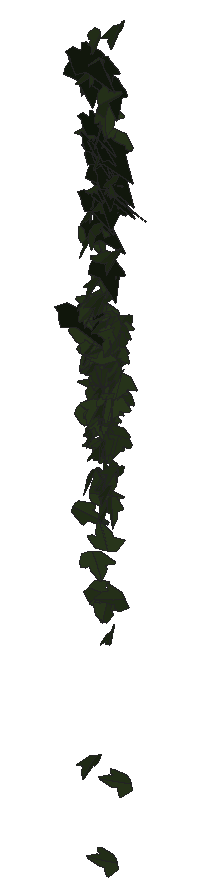
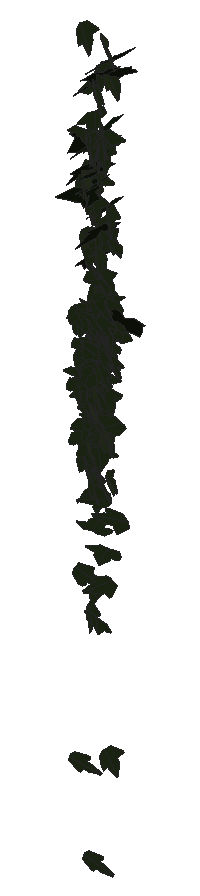
# SketchUp Ruby script. Lengths in inches.
U = 1.inch
M = Sketchup.active_model
def pt(a) = Geom::Point3d.new(a.map { |v| v * U })
def face(e, loops, mat)
  f = e.add_face(loops[0].map { |a| pt(a) })
  loops[1..].each { |l| e.add_face(l.map { |a| pt(a) }).erase! }
  f.material = f.back_material = mat if mat
  f
end
# faces: each face lists its corners as indices into pts; further lists are holes
def faces(e, pts, list, mat = nil) = list.each { |f| face(e, (f[0].is_a?(Array) ? f : [f]).map { |l| l.map { |i| pts[i] } }, mat) }
# xy, xz, yz: faces in a plane at the given z, y or x. An outline is a flat list of corners, or four numbers for a rectangle; further outlines are holes
def ring(l) = l.size == 4 ? [[l[0], l[1]], [l[2], l[1]], [l[2], l[3]], [l[0], l[3]]] : l.each_slice(2).to_a
def flat(e, list, mat, &to3) = list.each { |f| face(e, (f[0].is_a?(Array) ? f : [f]).map { |l| ring(l).map { |u, v| to3.(u, v) } }, mat) }
def xy(e, z, list, mat = nil) = flat(e, list, mat) { |x, y| [x, y, z] }
def xz(e, y, list, mat = nil) = flat(e, list, mat) { |x, z| [x, y, z] }
def yz(e, x, list, mat = nil) = flat(e, list, mat) { |y, z| [x, y, z] }
def lines(e, pts, list) = list.each { |a, b| e.add_line(pt(pts[a]), pt(pts[b])) }
# prism: a flat outline (further loops are holes) pulled along v
def prism(e, loops, v, mat = nil)
  f = face(e, loops, mat); d = Geom::Vector3d.new(v.map { |x| x * U })
  f.pushpull(f.normal.samedirection?(d) ? d.length : -d.length)
end
def box(e, o, s, mat = nil) = prism(e, [[o, [o[0] + s[0], o[1], o[2]], [o[0] + s[0], o[1] + s[1], o[2]], [o[0], o[1] + s[1], o[2]]]], [0, 0, s[2]], mat)
def at(x, y, z, deg = 0) = Geom::Transformation.translation(pt([x, y, z])) * Geom::Transformation.rotation(ORIGIN, Z_AXIS, deg.degrees)
def axes(o, x, y, z) = Geom::Transformation.new([*x, 0, *y, 0, *z, 0, *pt(o).to_a, 1])
def part(name) = M.definitions.add(name)
# library, detail: a bought-in or finely detailed component or shape, given as its bounding box
def library(name, o, s) = part(name).tap { |d| box(d.entities, o, s) }
def detail(e, o, s) = box(e.add_group.entities, o, s)
def put(e, d, t, mat = nil) = e.add_instance(d, t).tap { |i| i.material = mat if mat }
def group(e, t, mat = nil) = e.add_group.tap { |g| g.transformation = t; g.material = mat if mat }.entities
root = M.entities
M.materials.add("1026 AP 7946 SUNNY SIDE UP").color = [254, 231, 186]
M.materials.add("efeu1").color = [18, 25, 13]
M.materials.add("efeu2").color = [43, 57, 29]
c1 = part("ivyleaf_9")
p = [[1.54,2.16,1.25],[1.36,2.04,1.19],[-0.21,0.99,0.68],[-0.71,1.11,0.82],[-0.85,0.86,0.67],[-0.8,0.17,0.21],
  [-0.9,-0.01,0.1],[-0.67,-0.16,-0.02],[-0.08,-0.08,-0.05],[-0.03,-0.6,-0.4],[0.65,-0.88,-0.66],[0.83,-0.6,-0.49],
  [1.29,-0.42,-0.43],[1.8125,-0.07,-0.26],[1.21,0.44,0.15]]
faces(c1.entities,p,[[0,1,2,3,4,5,6,7,8,9,10,11,12,13,14]],"efeu1")
c2 = part("ivyleaf_10")
p = [[0,0.5,-0.03],[-0.0625,2.02,-0.43],[-0.19,2.01,-0.46],[-0.54,1.05,-0.29],[-0.52,0.625,-0.18],[-0.83,0.76,-0.28],
  [-1.16,0.64,-0.33],[-1.15,0.33,-0.24],[-0.77,-0.39,0.02],[-0.3,-0.51,0.16],[0.04,-0.48,0.23],[-0.02,2.01,-0.4375],
  [-0.06,2.01,-0.43],[0.04,-0.49,0.23],[0.67,-0.49,0.14],[1.38,0.36,-0.2],[1.375,0.51,-0.24],[0.81,0.65,-0.19],
  [0.62,0.59,-0.15],[0.6,1.09,-0.28],[0.5,1.23,-0.31]]
faces(c2.entities,p,[[0,1,2,3,4,5,6,7,8,9,10],[11,12,0,13,14,15,16,17,18,19,20]],"efeu2")
put(root,c1,axes([104.51,212.62,261.08],[-0.10189,-0.126,-0.22492],[0.26137,0.14715,-0.1379],[0.29668,-0.17291,0.04425]),"1026 AP 7946 SUNNY SIDE UP")
put(root,c2,axes([104.8,212.79,260.43],[0.14788,-0.18919,-0.06949],[-0.05325,0.05728,-0.21727],[0.31074,0.09986,-0.00416]),"1026 AP 7946 SUNNY SIDE UP")
put(root,c2,axes([104.78,212.86,258.33],[0.02808,-0.20182,0.05139],[-0.00344,-0.0514,-0.20892],[0.32731,0.01677,-0.00661]),"1026 AP 7946 SUNNY SIDE UP")
put(root,c2,axes([104.79,212.68,263.45],[0.03722,-0.22123,-0.10419],[-0.00875,0.09983,-0.22858],[0.38157,0.02387,0.00492]),"1026 AP 7946 SUNNY SIDE UP")
put(root,c2,axes([104.56,212.83,258.71],[0.15363,0.1008,0.18602],[0.18817,0.13453,-0.14375],[-0.26422,0.15442,0.00578]),"1026 AP 7946 SUNNY SIDE UP")
put(root,c2,axes([104.85,212.91,259.35],[-0.24055,-0.1247,0.08015],[-0.06584,-0.07172,-0.20183],[0.22216,-0.15628,0.02697]),"1026 AP 7946 SUNNY SIDE UP")
put(root,c2,axes([104.52,212.71,256.46],[-0.07971,-0.01702,-0.21016],[0.31895,-0.03174,-0.04941],[-0.04221,-0.2077,0.02353]),"1026 AP 7946 SUNNY SIDE UP")
put(root,c2,axes([104.81,212.76,260.13],[0.30669,-0.08194,-0.05742],[-0.09193,0.00295,-0.21702],[0.12532,0.2027,-0.01868]),"1026 AP 7946 SUNNY SIDE UP")
put(root,c2,axes([104.8125,212.65,266.57],[0.01044,-0.25506,0.02697],[-0.0004,-0.02764,-0.26301],[0.4034,0.00657,-0.00096]),"1026 AP 7946 SUNNY SIDE UP")
put(root,c2,axes([104.74,212.76,257.33],[0.11427,-0.15771,0.10792],[0.06501,-0.09726,-0.17944],[0.29132,0.08357,-0.00229]),"1026 AP 7946 SUNNY SIDE UP")
put(root,c2,axes([104.8,212.85,264.95],[0.0122,-0.23605,-0.05486],[0.0232,0.0523,-0.24244],[0.37933,0.00439,0.01659]),"1026 AP 7946 SUNNY SIDE UP")
put(root,c2,axes([104.79,212.67,262.84],[0.1113,-0.21199,0.07766],[0.02038,-0.07632,-0.2304],[0.35384,0.07108,-0.01116]),"1026 AP 7946 SUNNY SIDE UP")
put(root,c2,axes([104.83,212.74,258.55],[0.0412,-0.21263,-0.05682],[-0.02422,0.05241,-0.22022],[0.34408,0.02915,-0.0087]),"1026 AP 7946 SUNNY SIDE UP")
put(root,c2,axes([104.84,212.78,260.92],[0.22749,-0.13987,-0.09949],[-0.06758,0.09154,-0.20406],[0.25784,0.14739,0.03429]),"1026 AP 7946 SUNNY SIDE UP")
put(root,c2,axes([104.83,212.9,259.9],[-0.01707,-0.21632,0.02637],[0.00079,-0.02688,-0.22328],[0.34275,-0.01071,0.00183]),"1026 AP 7946 SUNNY SIDE UP")
put(root,c2,axes([104.91,212.97,259.98],[-0.30974,0.06925,0.05127],[-0.11245,-0.06746,-0.19686],[-0.07238,-0.19154,0.08646]),"1026 AP 7946 SUNNY SIDE UP")
put(root,c2,axes([104.82,212.81,267.33],[0.21445,-0.21888,-0.00563],[-0.01642,-0.00153,-0.2655],[0.34384,0.13644,-0.00916]),"1026 AP 7946 SUNNY SIDE UP")
put(root,c2,axes([104.89,212.73,261.34],[-0.14405,-0.16021,0.15164],[-0.034,-0.15318,-0.18537],[0.34138,-0.08286,0.04552]),"1026 AP 7946 SUNNY SIDE UP")
put(root,c2,axes([104.87,212.85,265.2],[-0.23667,-0.19164,0.0436],[0.00181,-0.05555,-0.24881],[0.30897,-0.14647,0.03486]),"1026 AP 7946 SUNNY SIDE UP")
put(root,c1,axes([104.72,212.6875,266.68],[-0.10214,-0.24221,-0.0535],[0.03916,0.04561,-0.25778],[0.38709,-0.06853,0.01196]),"1026 AP 7946 SUNNY SIDE UP")
put(root,c2,axes([104.875,212.9,259.69],[-0.22992,-0.14841,0.05033],[-0.00212,-0.06681,-0.21002],[0.24608,-0.13923,0.04521]),"1026 AP 7946 SUNNY SIDE UP")
put(root,c2,axes([104.85,212.67,260.38],[0.09904,-0.21439,0.04253],[0.00216,-0.04384,-0.23018],[0.34366,0.06206,-0.01081]),"1026 AP 7946 SUNNY SIDE UP")
put(root,c2,axes([104.74,213.15,254.29],[0.30393,-0.05318,0.06214],[0.08204,-0.03757,-0.20556],[0.09669,0.19906,-0.02091]),"1026 AP 7946 SUNNY SIDE UP")
put(root,c2,axes([104.88,212.64,250.91],[-0.04262,-0.21887,0.0626],[-0.01019,-0.06167,-0.22756],[0.35755,-0.02785,0.00097]),"1026 AP 7946 SUNNY SIDE UP")
put(root,c2,axes([104.83,212.73,261.375],[-0.13025,-0.20028,-0.08539],[0.0714,0.06949,-0.22238],[0.33256,-0.09336,0.0143]),"1026 AP 7946 SUNNY SIDE UP")
put(root,c2,axes([104.875,212.86,257.29],[0.18386,-0.17254,-0.02444],[-0.03716,0.0114,-0.21423],[0.27111,0.11857,-0.0128]),"1026 AP 7946 SUNNY SIDE UP")
put(root,c2,axes([104.875,212.62,261.21],[0.13267,-0.21299,-0.00805],[-0.01159,0.00418,-0.23592],[0.33486,0.08453,-0.00498]),"1026 AP 7946 SUNNY SIDE UP")
put(root,c2,axes([104.65,212.83,260.875],[0.2714,0.02668,0.13493],[0.20861,-0.01031,-0.17823],[-0.02353,0.21633,-0.02385]),"1026 AP 7946 SUNNY SIDE UP")
put(root,c2,axes([104.86,212.95,258.01],[-0.20099,-0.15647,0.02288],[0.04302,-0.05113,-0.2011],[0.24495,-0.11941,0.0541]),"1026 AP 7946 SUNNY SIDE UP")
put(root,c2,axes([104.8,212.77,258.53],[-0.05877,-0.11426,-0.19811],[0.11385,0.1776,-0.12259],[0.33187,-0.08116,0.00697]),"1026 AP 7946 SUNNY SIDE UP")
put(root,c2,axes([104.59,212.58,260.71],[0.13878,0.03307,0.21578],[0.32198,0.04486,-0.09601],[-0.08549,0.22264,-0.01132]),"1026 AP 7946 SUNNY SIDE UP")
put(root,c2,axes([104.89,212.91,260.31],[0.24752,-0.13403,-0.06789],[-0.05479,0.05902,-0.21151],[0.22783,0.15981,0.02289]),"1026 AP 7946 SUNNY SIDE UP")
put(root,c1,axes([104.67,212.58,267.03],[0.15689,-0.22817,-0.13244],[0.00758,0.13782,-0.24984],[0.41073,0.08461,0.0552]),"1026 AP 7946 SUNNY SIDE UP")
put(root,c1,axes([104.71,212.8,263.65],[0.14507,-0.22082,-0.04359],[0.00739,0.04627,-0.24525],[0.3531,0.08976,0.02304]),"1026 AP 7946 SUNNY SIDE UP")
put(root,c1,axes([104.72,212.78,264.99],[0.16245,-0.2222,-0.0096],[-0.01594,0.00416,-0.2523],[0.34926,0.10354,-0.00705]),"1026 AP 7946 SUNNY SIDE UP")
put(root,c2,axes([104.9375,212.88,262.53],[0.04453,-0.20147,-0.10635],[-0.01412,0.1018,-0.20894],[0.35486,0.02933,0.00503]),"1026 AP 7946 SUNNY SIDE UP")
put(root,c2,axes([104.7,212.82,262.87],[0.29867,0.00434,0.13971],[0.21332,-0.00654,-0.1956],[0.00042,0.23328,-0.00672]),"1026 AP 7946 SUNNY SIDE UP")
put(root,c2,axes([104.93,212.98,261.06],[0.37088,-0.00858,-0.06148],[-0.09463,-0.02243,-0.24203],[0.00438,0.24225,-0.02316]),"1026 AP 7946 SUNNY SIDE UP")
put(root,c2,axes([104.94,212.69,261.87],[0.02392,-0.21676,0.06373],[-0.00624,-0.06349,-0.22407],[0.35493,0.01349,-0.00824]),"1026 AP 7946 SUNNY SIDE UP")
put(root,c2,axes([104.92,212.97,261.44],[0.00887,-0.1694,0.14822],[0.03151,-0.14391,-0.17504],[0.34903,0.0173,0.01204]),"1026 AP 7946 SUNNY SIDE UP")
put(root,c2,axes([104.92,212.78,265.27],[0.16751,-0.2176,-0.0405],[0.00447,0.04362,-0.24836],[0.34733,0.10438,0.02273]),"1026 AP 7946 SUNNY SIDE UP")
put(root,c2,axes([105.02,212.9375,264.9],[-0.11881,0.18021,-0.14833],[-0.07566,0.13697,0.20199],[0.35576,0.08931,-0.00658]),"1026 AP 7946 SUNNY SIDE UP")
put(root,c2,axes([105.04,212.9375,264.89],[-0.0881,0.13873,-0.19698],[-0.10355,0.18039,0.15513],[0.35777,0.08637,-0.00361]),"1026 AP 7946 SUNNY SIDE UP")
put(root,c2,axes([104.95,212.9,259.4],[0.0345,-0.20898,-0.03506],[-0.00667,0.03258,-0.21628],[0.33257,0.02233,-0.0007]),"1026 AP 7946 SUNNY SIDE UP")
put(root,c2,axes([104.88,212.84,266.6875],[0.0196,-0.19245,0.17335],[0.10281,-0.16157,-0.19504],[0.38978,0.0523,0.04273]),"1026 AP 7946 SUNNY SIDE UP")
put(root,c2,axes([105.13,212.89,248.56],[0.10992,-0.04861,-0.19634],[-0.27901,0.07099,-0.08541],[0.13243,0.1899,-0.01699]),"1026 AP 7946 SUNNY SIDE UP")
put(root,c2,axes([104.9,212.84,260.68],[-0.15881,0.19158,-0.03443],[0.01209,-0.03492,-0.22311],[-0.30585,-0.10086,0.00906]),"1026 AP 7946 SUNNY SIDE UP")
put(root,c1,axes([104.74,212.74,265.47],[0.18142,-0.21141,-0.05815],[-0.01018,0.05914,-0.24672],[0.34343,0.11343,0.02341]),"1026 AP 7946 SUNNY SIDE UP")
put(root,c1,axes([104.81,212.91,266.73],[-0.03957,-0.24419,-0.04698],[0.03007,0.04241,-0.25221],[0.38905,-0.02812,0.01471]),"1026 AP 7946 SUNNY SIDE UP")
put(root,c2,axes([104.97,212.68,260.03],[-0.01743,-0.20268,-0.09054],[0.01155,0.08646,-0.20859],[0.34647,-0.01308,0.00239]),"1026 AP 7946 SUNNY SIDE UP")
put(root,c2,axes([104.97,212.7,258.99],[-0.14092,-0.1489,0.12829],[0.03546,-0.14504,-0.1617],[0.30402,-0.0521,0.07832]),"1026 AP 7946 SUNNY SIDE UP")
put(root,c2,axes([104.99,212.52,263.03],[0.00729,0.16944,0.16826],[-0.11423,0.15546,-0.16408],[-0.35088,-0.04709,0.05691]),"1026 AP 7946 SUNNY SIDE UP")
put(root,c2,axes([104.95,212.93,266.32],[0.23905,-0.19803,-0.02811],[0.01496,0.04002,-0.25488],[0.31373,0.14898,0.03357]),"1026 AP 7946 SUNNY SIDE UP")
put(root,c2,axes([104.96,212.7,259.79],[-0.13367,0.2056,0.00461],[-0.0107,0.00077,-0.22911],[-0.32315,-0.08507,0.00568]),"1026 AP 7946 SUNNY SIDE UP")
put(root,c1,axes([104.83,212.78,263.125],[0.12903,-0.16142,-0.18076],[-0.03745,0.17814,-0.18021],[0.37195,0.07393,0.04456]),"1026 AP 7946 SUNNY SIDE UP")
put(root,c2,axes([104.93,212.84,258.78],[0.30239,0.08387,0.00671],[-0.00149,0.01722,-0.2154],[-0.13222,0.19163,0.01777]),"1026 AP 7946 SUNNY SIDE UP")
put(root,c2,axes([105.08,212.82,258.66],[-0.21079,-0.12768,0.09723],[-0.06881,-0.08999,-0.18853],[0.24069,-0.13754,0.03125]),"1026 AP 7946 SUNNY SIDE UP")
put(root,c1,axes([104.85,212.86,264.86],[0.16655,-0.20467,-0.07825],[-0.07015,0.06103,-0.23679],[0.33539,0.11441,-0.01067]),"1026 AP 7946 SUNNY SIDE UP")
put(root,c2,axes([104.95,212.89,259.99],[0.17569,0.18057,-0.0365],[-0.01584,-0.03658,-0.2187],[-0.28922,0.11169,-0.01019]),"1026 AP 7946 SUNNY SIDE UP")
put(root,c2,axes([105.01,212.83,265.04],[0.15048,-0.21746,-0.05042],[0.01783,0.05663,-0.24212],[0.34961,0.09071,0.03405]),"1026 AP 7946 SUNNY SIDE UP")
put(root,c2,axes([105.04,212.69,264.86],[0.07104,-0.19852,-0.15328],[0.00097,0.15019,-0.20695],[0.38903,0.03588,0.02851]),"1026 AP 7946 SUNNY SIDE UP")
put(root,c2,axes([104.85,212.82,256.88],[0.01497,0.00423,0.20989],[0.1545,0.17857,-0.0075],[-0.28068,0.09852,0.00706]),"1026 AP 7946 SUNNY SIDE UP")
put(root,c2,axes([104.9375,212.73,258.72],[0.1286,0.19619,0.02211],[0.02398,0.01567,-0.21872],[-0.30921,0.08281,-0.00777]),"1026 AP 7946 SUNNY SIDE UP")
put(root,c2,axes([104.95,212.875,258.91],[0.31078,0.06482,0.03342],[0.0181,0.06394,-0.20585],[-0.11227,0.18975,0.05932]),"1026 AP 7946 SUNNY SIDE UP")
put(root,c2,axes([105.06,212.7,259.875],[-0.23693,-0.16871,-0.00416],[0.01977,-0.00712,-0.23262],[0.26459,-0.15055,0.01366]),"1026 AP 7946 SUNNY SIDE UP")
put(root,c2,axes([105.05,212.92,259.54],[-0.17262,-0.18301,-0.01059],[0.02551,0.00103,-0.21942],[0.287,-0.11017,0.01313]),"1026 AP 7946 SUNNY SIDE UP")
put(root,c2,axes([105.04,212.89,257.1875],[0.0108,-0.2003,0.02721],[0.0122,-0.02729,-0.20651],[0.31768,0.00785,0.00701]),"1026 AP 7946 SUNNY SIDE UP")
put(root,c2,axes([104.95,212.89,258.85],[0.13546,-0.14981,0.12258],[0.11621,-0.09531,-0.17803],[0.27837,0.11269,0.01467]),"1026 AP 7946 SUNNY SIDE UP")
put(root,c2,axes([105.07,212.9,259.89],[-0.17967,-0.18183,0.03669],[0.00996,-0.04685,-0.21936],[0.29148,-0.11048,0.03012]),"1026 AP 7946 SUNNY SIDE UP")
put(root,c2,axes([105.05,212.9,258.95],[0.10679,-0.19211,0.05494],[0.0072,-0.05597,-0.20976],[0.31389,0.06664,-0.01388]),"1026 AP 7946 SUNNY SIDE UP")
put(root,c2,axes([105.0625,212.61,258.12],[-0.01144,-0.20645,-0.08779],[0.0097,0.08387,-0.21231],[0.35036,-0.00907,0.00301]),"1026 AP 7946 SUNNY SIDE UP")
put(root,c2,axes([105.07,212.98,258.04],[-0.20275,-0.15391,0.02449],[0.02155,-0.04306,-0.20339],[0.24415,-0.12402,0.03829]),"1026 AP 7946 SUNNY SIDE UP")
put(root,c2,axes([105.0625,212.97,258.14],[0.05754,-0.19848,0.02598],[0.00192,-0.02656,-0.20804],[0.31482,0.03644,-0.00348]),"1026 AP 7946 SUNNY SIDE UP")
put(root,c2,axes([104.95,212.58,260.23],[0.3568,0.00702,-0.04494],[0.06621,0.03544,0.23152],[0.02125,-0.22834,0.03318]),"1026 AP 7946 SUNNY SIDE UP")
put(root,c2,axes([105.08,212.86,263.66],[-0.04251,-0.23699,-0.02156],[0.0164,0.01851,-0.24547],[0.37355,-0.02778,0.00832]),"1026 AP 7946 SUNNY SIDE UP")
put(root,c2,axes([105.05,212.92,260.16],[-0.34076,-0.01348,-0.02658],[0.04454,-0.05538,-0.21627],[0.01008,-0.21109,0.05711]),"1026 AP 7946 SUNNY SIDE UP")
put(root,c2,axes([105.09,212.66,261.54],[-0.11863,-0.23167,-0.03801],[0.0333,0.03049,-0.25059],[0.36705,-0.07764,0.01045]),"1026 AP 7946 SUNNY SIDE UP")
put(root,c2,axes([104.94,212.6,255.5625],[0.27316,0.10229,0.06261],[0.09265,0.0183,-0.20711],[-0.16201,0.18294,-0.01288]),"1026 AP 7946 SUNNY SIDE UP")
put(root,c2,axes([105.03,212.87,265.68],[0.11279,0.23045,-0.04043],[-0.03104,-0.0363,-0.24872],[-0.36662,0.07397,0.00862]),"1026 AP 7946 SUNNY SIDE UP")
put(root,c2,axes([104.93,212.62,254.84],[-0.10454,-0.08007,-0.18116],[0.22261,0.10568,-0.10436],[0.20581,-0.15497,0.02086]),"1026 AP 7946 SUNNY SIDE UP")
put(root,c2,axes([105.11,212.64,261.53],[0.03898,-0.22524,0.01485],[0.0002,-0.01577,-0.23352],[0.35502,0.02474,-0.0015]),"1026 AP 7946 SUNNY SIDE UP")
put(root,c2,axes([105.2,212.89,265.05],[0.06466,-0.1178,-0.21949],[-0.11747,0.19883,-0.12735],[0.36337,0.08524,-0.00211]),"1026 AP 7946 SUNNY SIDE UP")
put(root,c2,axes([105.13,212.9,260.96],[-0.08513,-0.20227,0.07095],[-0.01363,-0.07009,-0.21592],[0.3363,-0.05404,0.00921]),"1026 AP 7946 SUNNY SIDE UP")
put(root,c2,axes([105.1,212.8,259.07],[0.16096,-0.16881,-0.08013],[-0.00472,0.08623,-0.19882],[0.2916,0.09458,0.04101]),"1026 AP 7946 SUNNY SIDE UP")
put(root,c2,axes([105.19,212.8,260.33],[-0.01813,0.03336,-0.22057],[-0.18526,-0.18113,-0.02358],[-0.2863,0.11509,0.02922]),"1026 AP 7946 SUNNY SIDE UP")
put(root,c2,axes([104.87,212.64,261.04],[0.03226,0.05348,0.23743],[0.254,0.16545,-0.05347],[-0.27118,0.16132,-0.02184]),"1026 AP 7946 SUNNY SIDE UP")
put(root,c2,axes([105.16,212.68,257.49],[0.02001,-0.05498,-0.21489],[-0.03695,0.20704,-0.05657],[0.33669,0.02599,0.00656]),"1026 AP 7946 SUNNY SIDE UP")
put(root,c2,axes([105.01,212.91,259.81],[-0.10305,-0.14447,-0.14947],[0.17133,0.10339,-0.15704],[0.27149,-0.12008,0.04237]),"1026 AP 7946 SUNNY SIDE UP")
put(root,c2,axes([104.97,212.88,262.01],[0.29552,-0.07502,0.12556],[0.16388,-0.06715,-0.20781],[0.15506,0.21395,-0.01967]),"1026 AP 7946 SUNNY SIDE UP")
put(root,c2,axes([104.875,212.9,261.97],[0.22257,-0.01947,0.19434],[0.29031,-0.04025,-0.14715],[0.0689,0.23248,-0.00779]),"1026 AP 7946 SUNNY SIDE UP")
put(root,c2,axes([105.31,212.67,257.29],[0.1156,-0.00938,0.20537],[-0.29262,0.07367,0.07468],[-0.11358,-0.19935,0.01661]),"1026 AP 7946 SUNNY SIDE UP")
put(root,c2,axes([105.18,212.77,262.45],[-0.06378,-0.1995,0.1156],[-0.01755,-0.11325,-0.21013],[0.36036,-0.04082,0.01023]),"1026 AP 7946 SUNNY SIDE UP")
put(root,c2,axes([105.13,212.88,260.38],[-0.31699,-0.08579,-0.01638],[0.05599,-0.04562,-0.21854],[0.12509,-0.19697,0.05631]),"1026 AP 7946 SUNNY SIDE UP")
put(root,c2,axes([105.15,212.9,258.75],[0.1974,-0.16777,0.01334],[-0.00569,-0.02003,-0.21544],[0.26465,0.12471,-0.01458]),"1026 AP 7946 SUNNY SIDE UP")
put(root,c2,axes([105.19,212.88,258.49],[-0.31814,-0.05267,-0.00165],[0.00824,-0.01498,-0.21485],[0.08243,-0.20178,0.01511]),"1026 AP 7946 SUNNY SIDE UP")
put(root,c2,axes([105.18,212.6,259.14],[0.02568,-0.20498,-0.07419],[0.01855,0.07179,-0.21074],[0.34052,0.01155,0.01708]),"1026 AP 7946 SUNNY SIDE UP")
put(root,c1,axes([105.04,212.81,264.35],[-0.00843,-0.24643,-0.00181],[0.00607,0.00028,-0.25389],[0.38744,-0.00537,0.00394]),"1026 AP 7946 SUNNY SIDE UP")
put(root,c2,axes([105.1875,212.67,260.99],[-0.03399,-0.22196,-0.03471],[0.02203,0.03118,-0.22929],[0.35203,-0.02338,0.011]),"1026 AP 7946 SUNNY SIDE UP")
put(root,c2,axes([105.3125,212.59,260.5625],[-0.00362,-0.03156,-0.23191],[-0.1421,0.20651,-0.02769],[0.32767,0.0892,-0.01457]),"1026 AP 7946 SUNNY SIDE UP")
put(root,c2,axes([105.09,212.74,256.67],[-0.03048,0.01315,0.2144],[0.15874,-0.18221,0.02049],[0.28677,0.10226,0.01145]),"1026 AP 7946 SUNNY SIDE UP")
put(root,c2,axes([105.22,213,267.61],[-0.00953,-0.25298,0.01316],[0.01159,-0.01439,-0.26066],[0.39825,-0.00564,0.0079]),"1026 AP 7946 SUNNY SIDE UP")
put(root,c2,axes([105.3,212.82,263.6],[0.11947,-0.14206,-0.18129],[-0.12221,0.15703,-0.165],[0.33291,0.10862,0.00449]),"1026 AP 7946 SUNNY SIDE UP")
put(root,c2,axes([105.15,212.68,264.16],[-0.25151,0.15347,-0.09172],[0.05148,-0.09344,-0.22488],[-0.27489,-0.15792,0.0418]),"1026 AP 7946 SUNNY SIDE UP")
put(root,c2,axes([105.13,212.86,259.14],[-0.11933,0.14003,-0.1481],[0.05852,-0.14206,-0.16273],[-0.311,-0.08046,0.0262]),"1026 AP 7946 SUNNY SIDE UP")
put(root,c2,axes([105.26,212.69,264.0625],[-0.25506,-0.17485,0.01252],[0.00528,-0.021,-0.24523],[0.27567,-0.16138,0.01628]),"1026 AP 7946 SUNNY SIDE UP")
put(root,c2,axes([105.12,212.93,259.45],[0.32406,-0.01103,0.04566],[0.06773,-0.02202,-0.21182],[0.02417,0.20966,-0.0186]),"1026 AP 7946 SUNNY SIDE UP")
put(root,c2,axes([105.24,212.61,255.97],[0.28612,0.09224,0.04075],[-0.06921,0.00094,0.20913],[0.14147,-0.1861,0.0199]),"1026 AP 7946 SUNNY SIDE UP")
put(root,c1,axes([105.09,212.93,266.37],[0.01902,-0.24937,0.0265],[0.00211,-0.0271,-0.25736],[0.39441,0.01217,0.0001]),"1026 AP 7946 SUNNY SIDE UP")
put(root,c2,axes([105.34,212.5,258.1875],[0.16572,-0.07484,0.20769],[-0.23323,0.13791,0.13316],[-0.2457,-0.18139,0.01369]),"1026 AP 7946 SUNNY SIDE UP")
put(root,c2,axes([105.23,212.92,260.32],[0.3365,-0.03607,-0.03702],[-0.05709,-0.00052,-0.22348],[0.0558,0.21696,-0.00539]),"1026 AP 7946 SUNNY SIDE UP")
put(root,c2,axes([105.28,212.94,258.24],[-0.24869,-0.12152,0.03515],[-0.01714,-0.04243,-0.20389],[0.19802,-0.15628,0.02649]),"1026 AP 7946 SUNNY SIDE UP")
put(root,c2,axes([105.22,212.55,254.39],[0.05748,0.15433,-0.14493],[0.03805,0.13963,0.16407],[0.32708,-0.04336,0.00638]),"1026 AP 7946 SUNNY SIDE UP")
put(root,c2,axes([105.28,212.86,259.17],[-0.05846,-0.12149,0.17426],[-0.01844,-0.17103,-0.12968],[0.32784,-0.03129,0.02378]),"1026 AP 7946 SUNNY SIDE UP")
put(root,c2,axes([105.21,212.89,265.2],[0.38183,0.01343,-0.02645],[-0.03795,-0.02733,-0.24929],[-0.02541,0.24266,-0.02517]),"1026 AP 7946 SUNNY SIDE UP")
put(root,c1,axes([105.03,212.83,264.06],[0.19258,-0.20176,-0.06711],[0.02522,0.08257,-0.23608],[0.33188,0.11081,0.05688]),"1026 AP 7946 SUNNY SIDE UP")
put(root,c1,axes([105.08,212.74,265.04],[0.20707,-0.19051,-0.09589],[-0.05114,0.08885,-0.23698],[0.32871,0.13384,0.02354]),"1026 AP 7946 SUNNY SIDE UP")
put(root,c2,axes([105.28,212.66,257.25],[0.04701,-0.20214,0.03157],[0.00203,-0.03194,-0.21067],[0.32175,0.02974,-0.00328]),"1026 AP 7946 SUNNY SIDE UP")
put(root,c2,axes([105.28,212.84,260.1875],[-0.08863,-0.20591,-0.03955],[0.0293,0.03346,-0.21954],[0.32772,-0.05868,0.00893]),"1026 AP 7946 SUNNY SIDE UP")
put(root,c1,axes([105.18,212.7,262.32],[0.00414,-0.23851,-0.04106],[-0.00895,0.03843,-0.24545],[0.37979,0.00351,-0.00534]),"1026 AP 7946 SUNNY SIDE UP")
put(root,c2,axes([105.35,212.79,257.63],[-0.07251,-0.18868,0.06726],[-0.01509,-0.06593,-0.20039],[0.31414,-0.04672,0.0059]),"1026 AP 7946 SUNNY SIDE UP")
put(root,c2,axes([105.38,212.7,261.08],[0.23917,-0.14421,-0.09247],[-0.11566,0.05146,-0.21526],[0.23999,0.16852,-0.01159]),"1026 AP 7946 SUNNY SIDE UP")
put(root,c2,axes([105.26,212.9,264.05],[0.0799,-0.22749,0.05488],[0.08622,-0.0427,-0.23626],[0.35761,0.06112,0.0447]),"1026 AP 7946 SUNNY SIDE UP")
put(root,c2,axes([105.31,212.79,264.24],[0.07952,-0.21367,0.11606],[0.03647,-0.11152,-0.22683],[0.37895,0.05557,-0.00252]),"1026 AP 7946 SUNNY SIDE UP")
put(root,c2,axes([105.35,212.91,260.06],[-0.04039,-0.21406,0.03721],[-0.00364,-0.03732,-0.22231],[0.34165,-0.02571,0.00203]),"1026 AP 7946 SUNNY SIDE UP")
put(root,c2,axes([105.39,212.95,259.37],[-0.2995,0.07731,0.04856],[-0.0891,-0.01743,-0.2085],[-0.11059,-0.19534,0.03649]),"1026 AP 7946 SUNNY SIDE UP")
put(root,c1,axes([105.2,212.82,263.79],[-0.0366,-0.22468,0.09112],[0.0157,-0.09096,-0.23249],[0.38009,-0.01788,0.01838]),"1026 AP 7946 SUNNY SIDE UP")
put(root,c2,axes([105.29,212.76,259.2],[0.22279,0.14817,-0.06389],[-0.04841,-0.05725,-0.21085],[-0.24841,0.14405,-0.01621]),"1026 AP 7946 SUNNY SIDE UP")
put(root,c2,axes([105.3,212.82,260.73],[0.24329,-0.15663,0.03101],[0.03318,-0.02271,-0.22694],[0.24885,0.15615,-0.00006]),"1026 AP 7946 SUNNY SIDE UP")
put(root,c1,axes([105.13,212.69,264.99],[-0.0613,-0.14568,-0.20541],[0.19662,0.16148,-0.1464],[0.33361,-0.12195,0.04854]),"1026 AP 7946 SUNNY SIDE UP")
put(root,c2,axes([105.29,212.43,266.18],[0.00147,-0.01772,-0.27531],[0.11294,0.25736,-0.01582],[0.40554,-0.07161,0.0054]),"1026 AP 7946 SUNNY SIDE UP")
put(root,c2,axes([105.375,212.85,260.93],[-0.29371,0.11611,0.01198],[-0.04037,-0.02073,-0.22442],[-0.17889,-0.18596,0.03097]),"1026 AP 7946 SUNNY SIDE UP")
put(root,c1,axes([105.08,212.87,263.89],[0.31393,-0.13007,0.04457],[0.0837,0.00174,-0.24351],[0.19902,0.20443,0.03211]),"1026 AP 7946 SUNNY SIDE UP")
put(root,c2,axes([105.34,212.79,257.64],[0.19546,-0.16347,-0.00588],[0.02556,0.01832,-0.21],[0.25587,0.12304,0.02547]),"1026 AP 7946 SUNNY SIDE UP")
put(root,c1,axes([105.21,212.79,264.41],[0.08938,-0.20534,-0.12685],[-0.01366,0.12351,-0.21767],[0.37529,0.0534,0.02229]),"1026 AP 7946 SUNNY SIDE UP")
put(root,c2,axes([105.6,212.59,254.85],[-0.13436,0.00615,0.20078],[-0.29947,-0.04812,-0.08475],[0.06554,-0.20726,0.02436]),"1026 AP 7946 SUNNY SIDE UP")
put(root,c2,axes([105.39,212.56,254.03],[0.01246,-0.19052,-0.07474],[0.00844,0.07169,-0.19585],[0.31984,0.00553,0.00808]),"1026 AP 7946 SUNNY SIDE UP")
put(root,c2,axes([105.3,212.78,260.99],[0.20174,0.17874,-0.017],[-0.0001,-0.02148,-0.22643],[-0.2824,0.12769,-0.01206]),"1026 AP 7946 SUNNY SIDE UP")
put(root,c2,axes([105.33,212.93,259.66],[0.33096,0.02674,-0.00731],[-0.00742,-0.02007,-0.21779],[-0.04293,0.20965,-0.01866]),"1026 AP 7946 SUNNY SIDE UP")
put(root,c2,axes([105.43,212.91,261.05],[-0.11543,-0.20396,0.05757],[-0.01059,-0.05809,-0.22326],[0.33285,-0.07258,0.01286]),"1026 AP 7946 SUNNY SIDE UP")
put(root,c2,axes([105.33,212.7,256.91],[-0.01172,0.20916,-0.09346],[0.00724,-0.09181,-0.21614],[-0.35916,-0.00868,-0.0013]),"1026 AP 7946 SUNNY SIDE UP")
put(root,c2,axes([105.4,212.7,260.01],[0.235,-0.15627,-0.01278],[-0.0288,-0.00161,-0.22228],[0.24469,0.14989,-0.01388]),"1026 AP 7946 SUNNY SIDE UP")
put(root,c2,axes([105.45,212.73,260.76],[-0.14763,-0.17279,0.1313],[-0.01928,-0.1356,-0.19796],[0.33798,-0.08321,0.04606]),"1026 AP 7946 SUNNY SIDE UP")
put(root,c2,axes([105.6,212.73,250.6],[0.10227,-0.03885,-0.19401],[-0.28886,0.0454,-0.07483],[0.08817,0.19378,-0.02012]),"1026 AP 7946 SUNNY SIDE UP")
put(root,c2,axes([105.43,212.67,262.65],[0.01063,-0.23872,0.0334],[-0.00237,-0.03383,-0.24621],[0.37909,0.00648,-0.00248]),"1026 AP 7946 SUNNY SIDE UP")
put(root,c2,axes([105.41,212.8125,259.83],[0.02916,-0.20377,0.0744],[0.01193,-0.07299,-0.21122],[0.34034,0.02002,0.00103]),"1026 AP 7946 SUNNY SIDE UP")
